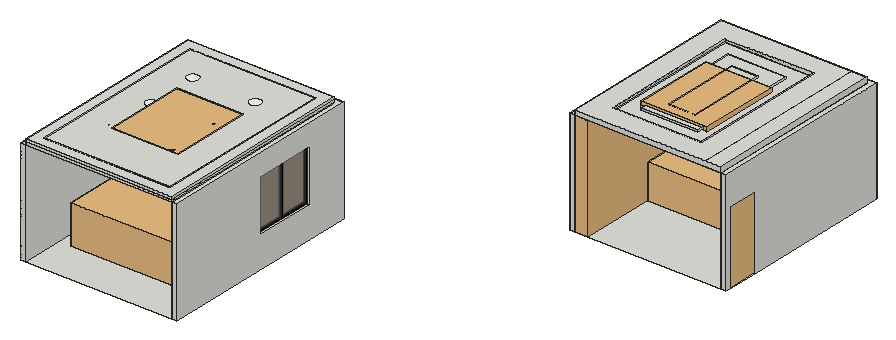
# SketchUp Ruby script. Lengths in inches.
U = 1.inch
M = Sketchup.active_model
def pt(a) = Geom::Point3d.new(a.map { |v| v * U })
def face(e, loops, mat)
  f = e.add_face(loops[0].map { |a| pt(a) })
  loops[1..].each { |l| e.add_face(l.map { |a| pt(a) }).erase! }
  f.material = f.back_material = mat if mat
  f
end
# faces: each face lists its corners as indices into pts; further lists are holes
def faces(e, pts, list, mat = nil) = list.each { |f| face(e, (f[0].is_a?(Array) ? f : [f]).map { |l| l.map { |i| pts[i] } }, mat) }
# xy, xz, yz: faces in a plane at the given z, y or x. An outline is a flat list of corners, or four numbers for a rectangle; further outlines are holes
def ring(l) = l.size == 4 ? [[l[0], l[1]], [l[2], l[1]], [l[2], l[3]], [l[0], l[3]]] : l.each_slice(2).to_a
def flat(e, list, mat, &to3) = list.each { |f| face(e, (f[0].is_a?(Array) ? f : [f]).map { |l| ring(l).map { |u, v| to3.(u, v) } }, mat) }
def xy(e, z, list, mat = nil) = flat(e, list, mat) { |x, y| [x, y, z] }
def xz(e, y, list, mat = nil) = flat(e, list, mat) { |x, z| [x, y, z] }
def yz(e, x, list, mat = nil) = flat(e, list, mat) { |y, z| [x, y, z] }
def lines(e, pts, list) = list.each { |a, b| e.add_line(pt(pts[a]), pt(pts[b])) }
# prism: a flat outline (further loops are holes) pulled along v
def prism(e, loops, v, mat = nil)
  f = face(e, loops, mat); d = Geom::Vector3d.new(v.map { |x| x * U })
  f.pushpull(f.normal.samedirection?(d) ? d.length : -d.length)
end
def box(e, o, s, mat = nil) = prism(e, [[o, [o[0] + s[0], o[1], o[2]], [o[0] + s[0], o[1] + s[1], o[2]], [o[0], o[1] + s[1], o[2]]]], [0, 0, s[2]], mat)
def at(x, y, z, deg = 0) = Geom::Transformation.translation(pt([x, y, z])) * Geom::Transformation.rotation(ORIGIN, Z_AXIS, deg.degrees)
def axes(o, x, y, z) = Geom::Transformation.new([*x, 0, *y, 0, *z, 0, *pt(o).to_a, 1])
def part(name) = M.definitions.add(name)
# library, detail: a bought-in or finely detailed component or shape, given as its bounding box
def library(name, o, s) = part(name).tap { |d| box(d.entities, o, s) }
def detail(e, o, s) = box(e.add_group.entities, o, s)
def put(e, d, t, mat = nil) = e.add_instance(d, t).tap { |i| i.material = mat if mat }
def group(e, t, mat = nil) = e.add_group.tap { |g| g.transformation = t; g.material = mat if mat }.entities
root = M.entities
M.materials.add("Plastic_Metalic_Black").color = [8, 8, 8]
M.materials.add("[Color M00]1").color = [254, 254, 254]
M.materials.add("[Color M00]2").color = [255, 255, 255]
M.materials.add("[Color M09]").color = [0, 0, 0]
M.materials.add("[Color_008]").color = [30, 30, 30]
M.materials.add("[Color_009]").color = [0, 0, 0]
M.materials.add("[Translucent_Glass_Gray]").color = [128, 128, 128]
M.materials["[Translucent_Glass_Gray]"].alpha = 0.5
c1 = library("Curtain set",[2.64,-2.53,0.02],[153.31,15.09,114.15])
c2 = library("sofa+(2)",[-100.93,-81.02,-0.06],[174.43,145.32,46.54])
c3 = part("Photos Gallery Wall")
g1 = group(c3.entities,at(0,0,0))
xy(g1,23.66,[[13.71,0.34,13.7,1.03,31.9375,1.12,31.94,0.43]],"Plastic_Metalic_Black")
xy(g1,24.66,[[14.71,0.34,30.94,0.42,30.9375,1.02,14.7,0.94]],"Plastic_Metalic_Black")
xy(g1,48.82,[[14.71,0.34,14.7,0.94,30.9375,1.02,30.94,0.42]],"Plastic_Metalic_Black")
xy(g1,49.82,[[13.71,0.34,31.94,0.43,31.9375,1.12,13.7,1.03]],"Plastic_Metalic_Black")
p = [[13.7,1.03,49.82],[13.7,1.03,23.66],[13.71,0.34,23.66],[13.71,0.34,49.82],[31.94,0.43,23.66],[31.94,0.43,49.82],
  [30.94,0.42,24.66],[14.71,0.34,24.66],[14.71,0.34,48.82],[30.94,0.42,48.82],[31.9375,1.12,23.66],[31.9375,1.12,49.82],
  [14.7,1.04,24.66],[30.9375,1.11,24.66],[30.9375,1.11,48.82],[14.7,1.04,48.82],[14.7,0.94,48.82],[14.7,0.94,24.66],
  [30.9375,1.02,24.66],[30.9375,1.02,48.82],[29.9375,1.02,47.82],[29.9375,1.02,25.66],[15.7,0.95,25.66],[15.7,0.95,47.82]]
faces(g1,p,[[0,1,2,3],[[4,5,3,2],[6,7,8,9]],[10,11,5,4],[[11,10,1,0],[12,13,14,15]],[16,8,7,17],[18,6,9,19],[21,20,23,22]],"Plastic_Metalic_Black")
faces(g1,p,[[[17,18,19,16],[20,21,22,23]]],"[Color M00]1")
lines(g1,p,[[14,19],[15,16],[12,17],[13,18]])
c4 = part("Photo+Frames+03")
put(c4.entities,c3,axes([128.61,79.32,-32.19],[1.3608,0,0],[0,1.3608,0],[0,0,1.3608]))
c5 = library("Round wall hanging",[0,0,0],[26.88,1.18,49.49])
c6 = library("ceiling fan",[0,0,0],[76.25,93.13,30.02])
c7 = library("main+door",[0,-0.79,0],[47.24,7.88,82.68])
c8 = library("Double bed",[0,0,0],[83.59,112.46,35.43])
c9 = library("Group\#1",[0,-1.58,0],[168,24.88,120])
c10 = part("Component\#5")
xy(c10.entities,0,[[6,0,7.55,0.2,9,0.8,10.24,1.76,11.2,3,11.8,4.45,12,6,11.8,7.55,11.2,9,10.24,10.24,9,11.2,7.55,11.8,6,12,4.45,11.8,3,11.2,1.76,10.24,0.8,9,0.2,7.55,0,6,0.2,4.45,0.8,3,1.76,1.76,3,0.8,4.45,0.2]],"[Color M00]1")
c11 = part("Square batten \#1")
box(c11.entities,[0,-1,0],[0.97,1,120])
c12 = part("Component\#7")
xy(c12.entities,0,[[4,0,5.04,0.14,6,0.54,6.83,1.17,7.46,2,7.86,2.96,8,4,7.86,5.04,7.46,6,6.83,6.83,6,7.46,5.04,7.86,4,8,2.96,7.86,2,7.46,1.17,6.83,0.54,6,0.14,5.04,0,4,0.14,2.96,0.54,2,1.17,1.17,2,0.54,2.96,0.14]],"[Color M00]2")
xy(root,0,[[6,0,174,234],[357.367,351.087,525.367,351.087,525.367,356.087,531.367,356.087,531.367,392.087,525.367,392.087,525.367,404.368,507.367,404.368,507.367,546.856,525.367,546.856,525.367,561.087,357.367,561.087]])
xy(root,6,[[507.367,404.368,525.367,404.368,525.367,546.856,507.547,546.856,507.547,428.116,507.367,428.116],[507.367,428.116,507.547,546.856]])
xy(root,6.2,[[507.367,428.316,507.547,451.664],[507.367,452.064,507.547,475.412],[507.367,475.812,507.547,499.16],[507.367,499.56,507.547,522.908],[507.367,523.308,507.547,546.656]])
xy(root,6.8,[[507.167,405.168,507.367,427.316]])
xy(root,17.059,[[507.167,405.168,507.367,427.316]])
xy(root,17.259,[[507.167,405.168,507.367,427.316]])
xy(root,27.075,[[507.167,405.168,507.367,427.316]])
xy(root,27.875,[[507.367,405.368,525.367,427.116]])
xy(root,36,[[174,118.8,180,190.8],[351.367,451.278,357.367,523.278]])
xy(root,47.25,[[507.367,405.368,525.367,427.116]])
xy(root,48.25,[[507.367,405.368,525.367,427.116]])
xy(root,67.625,[[507.367,405.368,525.367,427.116]])
xy(root,68.625,[[507.367,405.368,525.367,427.116]])
xy(root,84,[[525.367,356.087,531.367,392.087]])
xy(root,88.5,[[507.367,405.368,525.367,427.116]])
xy(root,89.3,[[507.367,428.316,507.547,451.664],[507.367,452.064,507.547,475.412],[507.367,475.812,507.547,499.16],[507.367,499.56,507.547,522.908],[507.367,523.308,507.547,546.656]])
xy(root,89.5,[[507.367,428.116,507.547,546.856]])
xy(root,90.5,[[507.367,404.368,507.547,546.856]])
xy(root,90.7,[[507.367,404.568,507.547,427.916],[507.367,428.316,507.547,451.664],[507.367,452.064,507.547,475.412],[507.367,475.812,507.547,499.16],[507.367,499.56,507.547,522.908],
  [507.367,523.308,507.547,546.656]])
xy(root,96,[[174,118.8,180,190.8],[351.367,451.278,357.367,523.278]])
xy(root,119.8,[[507.367,404.568,507.547,427.916],[507.367,428.316,507.547,451.664],[507.367,452.064,507.547,475.412],[507.367,475.812,507.547,499.16],[507.367,499.56,507.547,522.908],
  [507.367,523.308,507.547,546.656]])
xy(root,120,[[0,0,6,0,6,234,174,234,174,0,180,0,180,240,0,240],[351.367,351.087,357.367,351.087,357.367,561.087,525.367,561.087,525.367,351.087,531.367,351.087,531.367,567.087,351.367,567.087],[507.547,404.368,525.367,546.856]])
xz(root,0,[[0,0,6,120],[174,0,180,120]])
xz(root,118.8,[[174,36,180,96]])
xz(root,190.8,[[174,36,180,96]])
xz(root,234,[[6,0,174,120]])
xz(root,240,[[0,0,180,120]])
xz(root,351.087,[[351.367,0,357.367,120],[525.367,0,531.367,120]])
xz(root,356.087,[[525.367,0,531.367,84]])
xz(root,392.087,[[525.367,0,531.367,84]])
xz(root,404.368,[[507.367,0,525.367,6],[507.367,6,525.367,90],[507.367,90,525.367,90,525.367,120,507.547,120,507.547,90.5,507.367,90.5]])
xz(root,404.568,[[507.367,90.7,507.547,119.8]])
xz(root,405.168,[[507.167,6.8,507.367,17.059],[507.167,17.259,507.367,27.075]])
xz(root,405.368,[[507.367,27.875,525.367,47.25],[507.367,48.25,525.367,67.625],[507.367,68.625,525.367,88.5]])
xz(root,427.116,[[507.367,27.875,525.367,47.25],[507.367,48.25,525.367,67.625],[507.367,68.625,525.367,88.5]])
xz(root,427.316,[[507.167,6.8,507.367,17.059],[507.167,17.259,507.367,27.075]])
xz(root,427.916,[[507.367,90.7,507.547,119.8]])
xz(root,428.116,[[507.367,6,507.547,89.5]])
xz(root,428.316,[[507.367,6.2,507.547,89.3],[507.367,90.7,507.547,119.8]])
xz(root,451.278,[[351.367,36,357.367,96]])
xz(root,451.664,[[507.367,6.2,507.547,89.3],[507.367,90.7,507.547,119.8]])
xz(root,452.064,[[507.367,6.2,507.547,89.3],[507.367,90.7,507.547,119.8]])
xz(root,475.412,[[507.367,6.2,507.547,89.3],[507.367,90.7,507.547,119.8]])
xz(root,475.812,[[507.367,6.2,507.547,89.3],[507.367,90.7,507.547,119.8]])
xz(root,499.16,[[507.367,6.2,507.547,89.3],[507.367,90.7,507.547,119.8]])
xz(root,499.56,[[507.367,6.2,507.547,89.3],[507.367,90.7,507.547,119.8]])
xz(root,522.908,[[507.367,6.2,507.547,89.3],[507.367,90.7,507.547,119.8]])
xz(root,523.278,[[351.367,36,357.367,96]])
xz(root,523.308,[[507.367,6.2,507.547,89.3],[507.367,90.7,507.547,119.8]])
xz(root,546.656,[[507.367,6.2,507.547,89.3],[507.367,90.7,507.547,119.8]])
xz(root,546.856,[[507.367,0,525.367,6],[507.547,6,507.547,89.5,507.367,89.5,507.367,90,525.367,90,525.367,6],[507.367,90,507.367,90.5,507.547,90.5,507.547,120,525.367,120,525.367,90]])
xz(root,561.087,[[357.367,0,525.367,120]])
xz(root,567.087,[[351.367,0,531.367,120]])
yz(root,0,[[0,0,240,120]])
yz(root,6,[[0,0,234,120]])
yz(root,174,[[[0,0,234,120],[118.8,36,190.8,96]]])
yz(root,180,[[[0,0,240,120],[118.8,36,190.8,96]]])
yz(root,351.367,[[[351.087,0,567.087,120],[451.278,36,523.278,96]]])
yz(root,357.367,[[[351.087,0,561.087,120],[451.278,36,523.278,96]]])
yz(root,507.167,[[405.168,6.8,427.316,17.059],[405.168,17.259,427.316,27.075]])
yz(root,507.367,[[404.368,0,546.856,6],[[404.368,6,428.116,89.5],[405.368,27.875,427.116,67.625],[405.368,68.625,427.116,88.5],[405.168,6.8,427.316,17.059],[405.168,17.259,427.316,27.075]],[428.316,6.2,451.664,89.3],[452.064,6.2,475.412,89.3],[475.812,6.2,499.16,89.3],
  [499.56,6.2,522.908,89.3],[523.308,6.2,546.656,89.3],[405.368,47.25,427.116,48.25],[404.368,89.5,546.856,90.5],[404.568,90.7,427.916,119.8],
  [428.316,90.7,451.664,119.8],[452.064,90.7,475.412,119.8],[475.812,90.7,499.16,119.8],[499.56,90.7,522.908,119.8],[523.308,90.7,546.656,119.8]])
yz(root,507.547,[[[428.116,6,546.856,89.5],[428.316,6.2,451.664,89.3],[475.812,6.2,499.16,89.3],[499.56,6.2,522.908,89.3],[523.308,6.2,546.656,89.3],[452.064,6.2,475.412,89.3]],[[404.368,90.5,546.856,120],[428.316,90.7,451.664,119.8],[475.812,90.7,499.16,119.8],[404.568,90.7,427.916,119.8],[499.56,90.7,522.908,119.8],[523.308,90.7,546.656,119.8],[452.064,90.7,475.412,119.8]]])
yz(root,525.367,[[351.087,0,351.087,120,404.368,120,404.368,0,392.087,0,392.087,84,356.087,84,356.087,0],[546.856,0,561.087,120],[[404.368,6,546.856,90],[405.368,68.625,427.116,88.5],[405.368,48.25,427.116,67.625],[405.368,27.875,427.116,47.25]],[404.368,90,546.856,120]])
yz(root,531.367,[[351.087,0,351.087,120,567.087,120,567.087,0,392.087,0,392.087,84,356.087,84,356.087,0]])
p = [[66.562,-1210.213,541.354],[66.56,-1210.213,541.354],[66.56,-1210.213,540.318],[66.562,-1210.213,540.318],[641.791,-1212.5,407.959],[641.789,-1212.499,407.959],
  [641.789,-1212.499,406.923],[641.791,-1212.5,406.923]]
lines(root,p,[[0,1],[2,3],[4,5],[6,7]])
put(root,c1,axes([161.44,216.72,5.83],[0,-0.72,0],[1,0,0],[0,0,1]))
put(root,c2,axes([97.36,118.17,0.05],[0,-0.95666,0],[0.95666,0,0],[0,0,0.95666]))
put(root,c4,axes([93.16,307.35,48.29],[0,-1.45,0],[1,0,0],[0,0,1.35]))
put(root,c5,axes([18.46,228.49,69.94],[0.58039,0,0],[0,2.8,0],[0,0,0.64]))
put(root,c6,axes([53.64,64.42,103.49],[1,0,0],[0,1,0],[0,0,0.75]))
put(root,c7,axes([528.37,392.09,0],[0,-0.762,0],[0.25,0,0],[0,0,1.016]))
put(root,c8,axes([498.84,436.51,0],[0,1.12,0],[-1.12,0,0],[0,0,1.12]))
put(root,c1,axes([369.91,347.5,0],[0,1.36441,0],[-1,0,0],[0,0,1.05104]))
put(root,c9,at(6,209.5,0))
g2 = group(root,at(115.63,229.75,43.02,-180),"[Color M09]")
xy(g2,0,[[0,2,52.4375,4.5]])
xy(g2,12.7,[[19.25,0,34.44,2]])
xy(g2,20.57,[[19.25,0,34.44,2]])
xy(g2,32.125,[[0,2,52.4375,4.5]])
xz(g2,0,[[19.25,12.7,34.44,20.57]])
xz(g2,2,[[[0,0,52.4375,32.125],[19.25,12.7,34.44,20.57]]])
xz(g2,4.5,[[0,0,52.4375,32.125]])
yz(g2,0,[[2,0,4.5,32.125]])
yz(g2,19.25,[[0,12.7,2,20.57]])
yz(g2,34.44,[[0,12.7,2,20.57]])
yz(g2,52.4375,[[2,0,4.5,32.125]])
g3 = group(root,at(177.25,118.8,36))
xy(g3,0,[[-2.7,0,0,72]],"[Color_009]")
xy(g3,1.43,[[-2.7,1.71,-2.25,35.14],[-2.7,36.86,-2.25,70.29]])
xy(g3,1.43,[[-0.67,1.71,0,35.14],[-0.67,36.86,0,70.29]],"[Color_009]")
xy(g3,58.57,[[-2.7,1.71,-2.25,35.14],[-2.25,1.71,-0.67,35.14],[-0.67,1.71,0,35.14],[-2.7,36.86,-2.25,70.29],[-2.25,36.86,-0.67,70.29],
  [-0.67,36.86,0,70.29]])
xy(g3,60,[[-2.7,0,0,72]],"[Color_008]")
xz(g3,0,[[-2.7,0,0,60]],"[Color_009]")
xz(g3,1.71,[[-2.7,1.43,-2.25,58.57]])
xz(g3,1.71,[[-0.67,1.43,0,58.57]],"[Color_009]")
xz(g3,35.14,[[-2.7,1.43,-2.25,58.57],[-0.67,1.43,0,58.57]],"[Color_009]")
xz(g3,36.86,[[-2.7,1.43,-2.25,58.57],[-0.67,1.43,0,58.57]])
xz(g3,70.29,[[-2.7,1.43,-2.25,58.57],[-0.67,1.43,0,58.57]],"[Color_009]")
xz(g3,72,[[-2.7,0,0,60]],"[Color_009]")
yz(g3,-2.7,[[[0,0,72,60],[1.71,1.43,70.29,58.57]],[35.14,1.43,36.86,58.57]],"[Color_009]")
yz(g3,-2.25,[[1.71,1.43,35.14,58.57],[36.86,1.43,70.29,58.57]],"[Translucent_Glass_Gray]")
yz(g3,-0.67,[[1.71,1.43,35.14,58.57],[36.86,1.43,70.29,58.57]],"[Translucent_Glass_Gray]")
yz(g3,0,[[[0,0,72,60],[1.71,1.43,35.14,58.57],[36.86,1.43,70.29,58.57]]],"[Color_009]")
g4 = group(root,at(6,0,126))
xy(g4,-6,[[[0,0,168,234],[25,24,144,209]]])
xy(g4,-3,[[[0,0,168,234],[12,12,156,222]],[12,12,25,12,25,221,13,221,13,222,12,222],[25,12,144,24],[144,12,156,209],[25,209,156,209,156,222,13,222,13,221,25,221]])
xy(g4,0,[[[0,0,168,234],[12,12,156,222]],[12,12,156,222]])
xz(g4,0,[[0,-6,168,-3],[0,-3,168,0]])
xz(g4,12,[[12,-3,156,0]])
xz(g4,24,[[25,-6,144,-3]])
xz(g4,209,[[25,-6,144,-3]])
xz(g4,222,[[12,-3,156,0]])
xz(g4,234,[[0,-6,168,-3],[0,-3,168,0]])
yz(g4,0,[[0,-6,234,-3],[0,-3,234,0]])
yz(g4,12,[[12,-3,222,0]])
yz(g4,25,[[24,-6,209,-3]])
yz(g4,144,[[24,-6,209,-3]])
yz(g4,156,[[12,-3,222,0]])
yz(g4,168,[[0,-6,234,-3],[0,-3,234,0]])
put(g4,c10,axes([52.61,56.23,0],[-1,0,0],[0,1,0],[0,0,-1]))
put(g4,c10,axes([124.61,56.23,0],[-1,0,0],[0,1,0],[0,0,-1]))
put(g4,c10,axes([124.61,116.23,0],[-1,0,0],[0,1,0],[0,0,-1]))
put(g4,c10,axes([52.61,116.23,0],[-1,0,0],[0,1,0],[0,0,-1]))
put(g4,c10,axes([124.61,176.23,0],[-1,0,0],[0,1,0],[0,0,-1]))
put(g4,c10,axes([52.61,176.23,0],[-1,0,0],[0,1,0],[0,0,-1]))
g5 = group(root,at(357.37,559.28,0))
xy(g5,0,[[71,1,72,1.2],[95,1,96,1.2]])
xy(g5,120,[[71,1,72,1.2],[95,1,96,1.2]])
xz(g5,1,[[0.97,0,36,120],[36,0,48,120],[48,0,71,120],[72,0,95,120],[96,0,120,120],
  [120,0,132,120],[132,0,168,120]])
xz(g5,1.2,[[71,0,72,120],[95,0,96,120]])
yz(g5,71,[[1,0,1.2,120]])
yz(g5,72,[[1,0,1.2,120]])
yz(g5,95,[[1,0,1.2,120]])
yz(g5,96,[[1,0,1.2,120]])
put(g5,c11,at(135.6,1,0))
put(g5,c11,at(7.2,1,0))
put(g5,c11,at(12,1,0))
put(g5,c11,at(134.4,1,0))
put(g5,c11,at(3.6,1,0))
put(g5,c11,at(9.6,1,0))
put(g5,c11,at(138,1,0))
put(g5,c11,at(1.2,1,0))
put(g5,c11,at(10.8,1,0))
put(g5,c11,at(14.4,1,0))
put(g5,c11,at(28.8,1,0))
put(g5,c11,at(139.2,1,0))
put(g5,c11,at(24,1,0))
put(g5,c11,at(2.4,1,0))
put(g5,c11,at(30,1,0))
put(g5,c11,at(6,1,0))
put(g5,c11,at(22.8,1,0))
put(g5,c11,at(32.4,1,0))
put(g5,c11,at(136.8,1,0))
put(g5,c11,at(16.8,1,0))
put(g5,c11,at(4.8,1,0))
put(g5,c11,at(15.6,1,0))
put(g5,c11,at(133.2,1,0))
put(g5,c11,at(140.4,1,0))
put(g5,c11,at(27.6,1,0))
put(g5,c11,at(26.4,1,0))
put(g5,c11,at(31.2,1,0))
put(g5,c11,at(25.2,1,0))
put(g5,c11,at(132,1,0))
put(g5,c11,at(8.4,1,0))
put(g5,c11,at(13.2,1,0))
put(g5,c11,at(20.4,1,0))
put(g5,c11,at(18,1,0))
put(g5,c11,at(21.6,1,0))
put(g5,c11,at(33.6,1,0))
put(g5,c11,at(34.8,1,0))
put(g5,c11,at(19.2,1,0))
put(g5,c11,at(151.2,1,0))
put(g5,c11,at(142.8,1,0))
put(g5,c11,at(156,1,0))
put(g5,c11,at(157.2,1,0))
put(g5,c11,at(158.4,1,0))
put(g5,c11,at(147.6,1,0))
put(g5,c11,at(159.6,1,0))
put(g5,c11,at(144,1,0))
put(g5,c11,at(154.8,1,0))
put(g5,c11,at(153.6,1,0))
put(g5,c11,at(150,1,0))
put(g5,c11,at(160.8,1,0))
put(g5,c11,at(166.8,1,0))
put(g5,c11,at(162,1,0))
put(g5,c11,at(146.4,1,0))
put(g5,c11,at(164.4,1,0))
put(g5,c11,at(141.6,1,0))
put(g5,c11,at(145.2,1,0))
put(g5,c11,at(152.4,1,0))
put(g5,c11,at(148.8,1,0))
put(g5,c11,at(163.2,1,0))
put(g5,c11,at(165.6,1,0))
put(g5,c11,at(0,1,0))
g6 = group(root,at(355.03,451.28,36))
xy(g6,0,[[-2.34,0,0,72]],"[Color_009]")
xy(g6,1.43,[[-2.34,1.71,-1.95,35.14],[-2.34,36.86,-1.95,70.29]])
xy(g6,1.43,[[-0.58,1.71,0,35.14],[-0.58,36.86,0,70.29]],"[Color_009]")
xy(g6,58.57,[[-2.34,1.71,-1.95,35.14],[-1.95,1.71,-0.58,35.14],[-0.58,1.71,0,35.14],[-2.34,36.86,-1.95,70.29],[-1.95,36.86,-0.58,70.29],
  [-0.58,36.86,0,70.29]])
xy(g6,60,[[-2.34,0,0,72]],"[Color_008]")
xz(g6,0,[[-2.34,0,0,60]],"[Color_009]")
xz(g6,1.71,[[-2.34,1.43,-1.95,58.57]])
xz(g6,1.71,[[-0.58,1.43,0,58.57]],"[Color_009]")
xz(g6,35.14,[[-2.34,1.43,-1.95,58.57],[-0.58,1.43,0,58.57]],"[Color_009]")
xz(g6,36.86,[[-2.34,1.43,-1.95,58.57],[-0.58,1.43,0,58.57]])
xz(g6,70.29,[[-2.34,1.43,-1.95,58.57],[-0.58,1.43,0,58.57]],"[Color_009]")
xz(g6,72,[[-2.34,0,0,60]],"[Color_009]")
yz(g6,-2.34,[[[0,0,72,60],[1.71,1.43,70.29,58.57]],[35.14,1.43,36.86,58.57]],"[Color_009]")
yz(g6,-1.95,[[1.71,1.43,35.14,58.57],[36.86,1.43,70.29,58.57]],"[Translucent_Glass_Gray]")
yz(g6,-0.58,[[1.71,1.43,35.14,58.57],[36.86,1.43,70.29,58.57]],"[Translucent_Glass_Gray]")
yz(g6,0,[[[0,0,72,60],[1.71,1.43,35.14,58.57],[36.86,1.43,70.29,58.57]]],"[Color_009]")
g7 = group(root,at(357.37,351.09,99.89))
p = [[150.18,0,26.11],[150.18,53.28,26.11],[150.18,210,26.11]]
lines(g7,p,[[0,1],[1,2]])
put(g7,c6,axes([37.08,48.7,0],[1,0,0],[0,1,0],[0,0,0.87]))
g8 = group(g7,at(0,0,26.11))
xy(g8,-6,[[[0,0,168,210],[24,24,126.18,186]]])
xy(g8,-4,[[[24,24,126.18,186],[42,42,108.18,168]]])
xy(g8,-2,[[[42,42,108.18,168],[60,60,90.18,150]]])
xy(g8,0,[[[0,0,168,210],[24,24,126.18,186]],[60,60,90.18,150]])
xz(g8,0,[[0,-6,168,0]])
xz(g8,24,[[24,-6,126.18,-4],[24,-4,126.18,0]])
xz(g8,42,[[42,-4,108.18,-2]])
xz(g8,60,[[60,-2,90.18,0]])
xz(g8,150,[[60,-2,90.18,0]])
xz(g8,168,[[42,-4,108.18,-2]])
xz(g8,186,[[24,-6,126.18,-4],[24,-4,126.18,0]])
xz(g8,210,[[0,-6,168,0]])
yz(g8,0,[[0,-6,210,0]])
yz(g8,24,[[24,-6,186,-4],[24,-4,186,0]])
yz(g8,42,[[42,-4,168,-2]])
yz(g8,60,[[60,-2,150,0]])
yz(g8,90.18,[[60,-2,150,0]])
yz(g8,108.18,[[42,-4,168,-2]])
yz(g8,126.18,[[24,-6,186,-4],[24,-4,186,0]])
yz(g8,168,[[0,-6,210,0]])
put(g8,c12,axes([16.57,38.05,-6],[-1,0,0],[0,1,0],[0,0,-1]))
put(g8,c12,axes([140.01,38.05,-6],[-1,0,0],[0,1,0],[0,0,-1]))
put(g8,c12,axes([16.57,164.55,-6],[-1,0,0],[0,1,0],[0,0,-1]))
put(g8,c12,axes([140.01,164.55,-6],[-1,0,0],[0,1,0],[0,0,-1]))
put(g8,c12,axes([140.01,125.42,-6],[-1,0,0],[0,1,0],[0,0,-1]))
put(g8,c12,axes([16.57,125.42,-6],[-1,0,0],[0,1,0],[0,0,-1]))
put(g8,c12,axes([16.57,81.3,-6],[-1,0,0],[0,1,0],[0,0,-1]))
put(g8,c12,axes([140.01,81.3,-6],[-1,0,0],[0,1,0],[0,0,-1]))
put(g8,c12,axes([43.42,7.64,-6],[-1,0,0],[0,1,0],[0,0,-1]))
put(g8,c12,axes([109.67,7.64,-6],[-1,0,0],[0,1,0],[0,0,-1]))
put(g8,c12,axes([43.42,194.39,-6],[-1,0,0],[0,1,0],[0,0,-1]))
put(g8,c12,axes([109.67,194.39,-6],[-1,0,0],[0,1,0],[0,0,-1]),"[Color M00]2")
